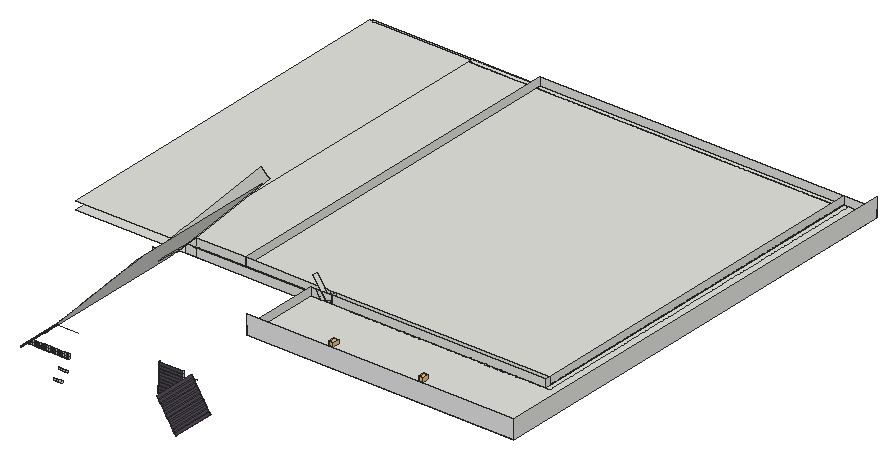
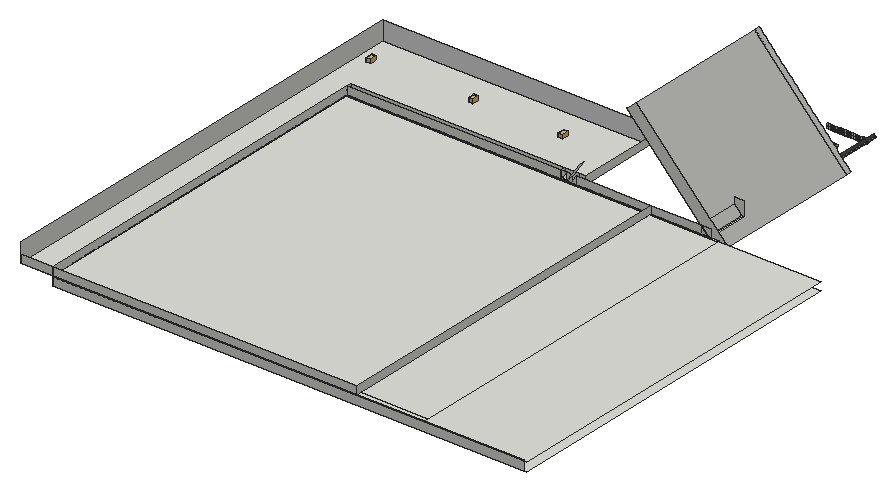
# SketchUp Ruby script. Lengths in inches.
U = 1.inch
M = Sketchup.active_model
def pt(a) = Geom::Point3d.new(a.map { |v| v * U })
def face(e, loops, mat)
  f = e.add_face(loops[0].map { |a| pt(a) })
  loops[1..].each { |l| e.add_face(l.map { |a| pt(a) }).erase! }
  f.material = f.back_material = mat if mat
  f
end
# faces: each face lists its corners as indices into pts; further lists are holes
def faces(e, pts, list, mat = nil) = list.each { |f| face(e, (f[0].is_a?(Array) ? f : [f]).map { |l| l.map { |i| pts[i] } }, mat) }
# xy, xz, yz: faces in a plane at the given z, y or x. An outline is a flat list of corners, or four numbers for a rectangle; further outlines are holes
def ring(l) = l.size == 4 ? [[l[0], l[1]], [l[2], l[1]], [l[2], l[3]], [l[0], l[3]]] : l.each_slice(2).to_a
def flat(e, list, mat, &to3) = list.each { |f| face(e, (f[0].is_a?(Array) ? f : [f]).map { |l| ring(l).map { |u, v| to3.(u, v) } }, mat) }
def xy(e, z, list, mat = nil) = flat(e, list, mat) { |x, y| [x, y, z] }
def xz(e, y, list, mat = nil) = flat(e, list, mat) { |x, z| [x, y, z] }
def yz(e, x, list, mat = nil) = flat(e, list, mat) { |y, z| [x, y, z] }
def lines(e, pts, list) = list.each { |a, b| e.add_line(pt(pts[a]), pt(pts[b])) }
# prism: a flat outline (further loops are holes) pulled along v
def prism(e, loops, v, mat = nil)
  f = face(e, loops, mat); d = Geom::Vector3d.new(v.map { |x| x * U })
  f.pushpull(f.normal.samedirection?(d) ? d.length : -d.length)
end
def box(e, o, s, mat = nil) = prism(e, [[o, [o[0] + s[0], o[1], o[2]], [o[0] + s[0], o[1] + s[1], o[2]], [o[0], o[1] + s[1], o[2]]]], [0, 0, s[2]], mat)
def at(x, y, z, deg = 0) = Geom::Transformation.translation(pt([x, y, z])) * Geom::Transformation.rotation(ORIGIN, Z_AXIS, deg.degrees)
def axes(o, x, y, z) = Geom::Transformation.new([*x, 0, *y, 0, *z, 0, *pt(o).to_a, 1])
def part(name) = M.definitions.add(name)
# library, detail: a bought-in or finely detailed component or shape, given as its bounding box
def library(name, o, s) = part(name).tap { |d| box(d.entities, o, s) }
def detail(e, o, s) = box(e.add_group.entities, o, s)
def put(e, d, t, mat = nil) = e.add_instance(d, t).tap { |i| i.material = mat if mat }
def group(e, t, mat = nil) = e.add_group.tap { |g| g.transformation = t; g.material = mat if mat }.entities
root = M.entities
M.materials.add("[Color M01]").color = [226, 226, 226]
M.materials.add("[Color M06]").color = [79, 71, 84]
c1 = library("Group\#13",[0,0,0],[3.54,3.54,3.9375])
xy(root,306.39,[[2350.98,523.75,2381.95,526.125]])
xy(root,307.2,[[2350.98,523.75,2381.95,526.125]])
xy(root,310.33,[[2350.98,523.75,2381.95,526.125]])
xy(root,311.14,[[2350.98,523.75,2381.95,526.125]])
xy(root,314.27,[[2350.98,523.75,2381.95,526.125]])
xy(root,315.08,[[2350.98,524.25,2381.95,526.125]])
xy(root,318.2,[[2350.98,524.25,2381.95,526.125]])
xy(root,319.01,[[2350.98,524.25,2381.95,526.125]])
xy(root,322.14,[[2350.98,524.25,2381.95,526.125]])
xy(root,322.89,[[2350.98,524.25,2381.95,526.125]])
xy(root,326.02,[[2350.98,524.25,2381.95,526.125]])
xy(root,326.76,[[2350.98,524.25,2381.95,526.125]])
xy(root,328,[[2079.13,732.2,2683.5,1201.875]])
xy(root,329.89,[[2350.98,524.25,2381.95,526.125]])
xy(root,330.64,[[2350.98,524.25,2381.95,526.125]])
xy(root,333.77,[[2350.98,524.25,2381.95,526.125]])
xy(root,334.51,[[2350.98,524.25,2381.95,526.125]])
xy(root,336.02,[[2220.6875,480.14,2223,480.77],[2223.6,480.14,2225.91,480.77],[2226.51,480.14,2228.82,480.77],[2229.42,480.14,2231.73,480.77],[2232.33,480.14,2234.65,480.77],
  [2235.25,480.14,2237.56,480.77],[2238.16,480.14,2240.47,480.77],[2241.07,480.14,2243.38,480.77],[2243.98,480.14,2246.29,480.77],[2246.89,480.14,2249.21,480.77],
  [2249.81,480.14,2252.12,480.77],[2252.72,480.14,2255.03,480.77],[2255.63,480.14,2257.94,480.77],[2258.54,480.14,2260.86,480.77],[2261.45,480.14,2263.77,480.77],
  [2264.37,480.14,2266.68,480.77],[2267.28,480.14,2269.59,480.77],[2270.19,480.14,2272.5,480.77]])
xy(root,336.52,[[2220.6875,480.14,2223,480.77],[2223.6,480.14,2225.91,480.77],[2226.51,480.14,2228.82,480.77],[2229.42,480.14,2231.73,480.77],[2232.33,480.14,2234.65,480.77],
  [2235.25,480.14,2237.56,480.77],[2238.16,480.14,2240.47,480.77],[2241.07,480.14,2243.38,480.77],[2243.98,480.14,2246.29,480.77],[2246.89,480.14,2249.21,480.77],
  [2249.81,480.14,2252.12,480.77],[2252.72,480.14,2255.03,480.77],[2255.63,480.14,2257.94,480.77],[2258.54,480.14,2260.86,480.77],[2261.45,480.14,2263.77,480.77],
  [2264.37,480.14,2266.68,480.77],[2267.28,480.14,2269.59,480.77],[2270.19,480.14,2272.5,480.77]])
xy(root,337.64,[[2350.98,524.25,2381.95,526.125]])
xy(root,338.39,[[2350.98,524.25,2381.95,526.125]])
xy(root,338.84,[[2222.47,480.14,2223,480.77],[2223.6,480.14,2225.91,480.77],[2226.51,480.14,2228.82,480.77],[2229.42,480.14,2231.73,480.77],[2232.33,480.14,2234.65,480.77],
  [2235.25,480.14,2237.56,480.77],[2238.16,480.14,2240.47,480.77],[2241.07,480.14,2243.38,480.77],[2243.98,480.14,2246.29,480.77],[2246.89,480.14,2249.21,480.77],
  [2249.81,480.14,2252.12,480.77],[2252.72,480.14,2255.03,480.77],[2255.63,480.14,2257.94,480.77],[2258.54,480.14,2260.86,480.77],[2261.45,480.14,2263.77,480.77],
  [2264.37,480.14,2266.68,480.77],[2267.28,480.14,2269.59,480.77],[2270.19,480.14,2272.5,480.77]])
xy(root,338.875,[[2079.13,732.2,2683.5,1201.875]])
xy(root,339.34,[[2223.6,480.14,2225.91,480.77],[2226.51,480.14,2228.82,480.77],[2229.42,480.14,2231.73,480.77],[2232.33,480.14,2234.65,480.77],[2235.25,480.14,2237.56,480.77],
  [2238.16,480.14,2240.47,480.77],[2241.07,480.14,2243.38,480.77],[2243.98,480.14,2246.29,480.77],[2246.89,480.14,2249.21,480.77],[2249.81,480.14,2252.12,480.77],
  [2252.72,480.14,2255.03,480.77],[2255.63,480.14,2257.94,480.77],[2258.54,480.14,2260.86,480.77],[2261.45,480.14,2263.77,480.77],[2264.37,480.14,2266.68,480.77],
  [2267.28,480.14,2269.59,480.77],[2270.19,480.14,2272.5,480.77]])
xy(root,340.125,[[2384.28,623.84,2384.28,726.125,2436.62,726.125,2436.62,724.8125,2442.7,724.8125,2442.7,726.125,2446.12,726.125,2446.12,724.8125,2452.2,724.8125,2452.2,726.125,2455.62,726.125,2455.62,724.8125,2461.7,724.8125,2461.7,726.125,2465.12,726.125,2465.12,724.8125,2471.2,724.8125,2471.2,726.125,2474.62,726.125,2474.62,724.8125,2480.7,724.8125,2480.7,726.125,2484.12,726.125,2484.12,724.8125,2490.2,724.8125,2490.2,726.125,2493.62,726.125,2493.62,724.8125,2499.7,724.8125,2499.7,726.125,2503.12,726.125,2503.12,724.8125,2509.2,724.8125,2509.2,726.125,2512.62,726.125,2512.62,724.8125,2518.7,724.8125,2518.7,726.125,2522.12,726.125,2522.12,724.8125,2528.2,724.8125,2528.2,726.125,2531.62,726.125,2531.62,724.8125,2537.7,724.8125,2537.7,726.125,2541.12,726.125,2541.12,724.8125,2547.2,724.8125,2547.2,726.125,2550.62,726.125,2550.62,724.8125,2556.7,724.8125,2556.7,726.125,2560.12,726.125,2560.12,724.8125,2566.2,724.8125,2566.2,726.125,2569.62,726.125,2569.62,724.8125,2575.7,724.8125,2575.7,726.125,2579.12,726.125,2579.12,724.8125,2585.2,724.8125,2585.2,726.125,2588.62,726.125,2588.62,724.8125,2594.7,724.8125,2594.7,726.125,2598.12,726.125,2598.12,724.8125,2604.2,724.8125,2604.2,726.125,2607.62,726.125,2607.62,724.8125,2613.7,724.8125,2613.7,726.125,2617.12,726.125,2617.12,724.8125,2623.2,724.8125,2623.2,726.125,2626.62,726.125,2626.62,724.8125,2632.7,724.8125,2632.7,726.125,2636.12,726.125,2636.12,724.8125,2642.2,724.8125,2642.2,726.125,2645.62,726.125,2645.62,724.8125,2651.7,724.8125,2651.7,726.125,2655.12,726.125,2655.12,724.8125,2661.2,724.8125,2661.2,726.125,2664.62,726.125,2664.62,724.8125,2670.7,724.8125,2670.7,726.125,2674.12,726.125,2674.12,724.8125,2680.2,724.8125,2680.2,726.125,2683.62,726.125,2683.62,724.8125,2689.7,724.8125,2689.7,1201.875,2724.93,1201.875,2724.93,623.84],[2219.8,678.64,2222.65,726.125],[2436.62,724.8125,2442.7,726.125],[2446.12,724.8125,2452.2,726.125],[2455.62,724.8125,2461.7,726.125],
  [2465.12,724.8125,2471.2,726.125],[2474.62,724.8125,2480.7,726.125],[2484.12,724.8125,2490.2,726.125],[2493.62,724.8125,2499.7,726.125],[2503.12,724.8125,2509.2,726.125],
  [2512.62,724.8125,2518.7,726.125],[2522.12,724.8125,2528.2,726.125],[2531.62,724.8125,2537.7,726.125],[2541.12,724.8125,2547.2,726.125],[2550.62,724.8125,2556.7,726.125],
  [2560.12,724.8125,2566.2,726.125],[2569.62,724.8125,2575.7,726.125],[2579.12,724.8125,2585.2,726.125],[2588.62,724.8125,2594.7,726.125],[2598.12,724.8125,2604.2,726.125],
  [2607.62,724.8125,2613.7,726.125],[2617.12,724.8125,2623.2,726.125],[2626.62,724.8125,2632.7,726.125],[2636.12,724.8125,2642.2,726.125],[2645.62,724.8125,2651.7,726.125],
  [2655.12,724.8125,2661.2,726.125],[2664.62,724.8125,2670.7,726.125],[2674.12,724.8125,2680.2,726.125],[2683.62,724.8125,2689.7,1201.875],[2219.8,726.125,2222.65,732.2],
  [2410.35,726.125,2683.5,732.2],[2683.5,726.125,2683.62,732.2],[2209.43,732.2,2295.55,734.4375],[2295.55,732.2,2410.35,734.4375],[2410.35,732.2,2683.5,734.4375],
  [2683.5,732.2,2683.62,734.4375],[2209.43,734.4375,2295.55,1195.68],[2295.55,734.4375,2683.5,1195.68],[2683.5,734.4375,2683.62,1195.8],[2209.43,1195.68,2295.55,1195.8],
  [2295.55,1195.68,2683.5,1195.8],[2209.43,1195.8,2295.55,1201.875],[2295.55,1195.8,2683.5,1201.875],[2683.5,1195.8,2683.62,1201.875]])
xz(root,480.64,[[2252.6875,305.35,2255,307.67],[2255.6,305.35,2257.91,307.67],[2258.51,305.35,2260.83,307.67],[2261.43,305.35,2263.74,307.67]])
xz(root,480.7,[[2258.54,319.65,2260.86,321.96],[2261.45,319.65,2263.77,321.96],[2264.37,319.65,2266.68,321.96],[2267.28,319.65,2269.59,321.96]])
xz(root,521.5625,[[2419,305.32,2419.37,305.56,2417.67,308.2,2417.3,307.97],[2416.77,308.8,2417.14,309.03,2415.44,311.68,2415.08,311.44],[2414.54,312.27,2414.91,312.51,2413.22,315.15,2412.85,314.91],[2412.32,315.74,2412.6875,315.98,2410.99,318.62,2410.625,318.38],[2410.09,319.21,2410.46,319.45,2408.77,322.09,2408.4,321.86],
  [2407.87,322.6875,2408.23,322.92,2406.54,325.57,2406.17,325.33],[2405.64,326.16,2406.01,326.4,2404.3125,329.04,2403.94,328.8],[2403.41,329.63,2403.78,329.87,2402.09,332.51,2401.72,332.28],[2401.1875,333.11,2401.55,333.34,2399.86,335.98,2399.49,335.75],[2398.96,336.58,2399.33,336.8125,2397.63,339.46,2397.27,339.22],
  [2221.68,338.19,2223.1,339.7,2222.65,340.125,2221.23,338.62],[2223.1,339.7,2223.5,340.125,2222.65,340.125],[2396.73,340.05,2397.1,340.29,2395.41,342.93,2395.04,342.69],[2222.65,340.125,2223.5,340.125,2224.11,340.76,2223.65,341.19]])
xz(root,523.75,[[2350.98,307.2,2381.95,310.33],[2350.98,311.14,2381.95,314.27]],"[Color M06]")
xz(root,524.25,[[2350.98,315.08,2381.95,318.2],[2350.98,319.01,2381.95,322.14],[2350.98,322.89,2381.95,326.02],[2350.98,326.76,2381.95,329.89],[2350.98,330.64,2381.95,333.77],
  [2350.98,334.51,2381.95,337.64],[2350.98,338.39,2381.95,341.52]],"[Color M06]")
xz(root,526.125,[[2350.98,306.39,2381.95,307.2],[2350.98,310.33,2381.95,311.14],[2350.98,314.27,2381.95,315.08],[2350.98,318.2,2381.95,319.01],[2350.98,322.14,2381.95,322.89],
  [2350.98,326.02,2381.95,326.76],[2350.98,329.89,2381.95,330.64],[2350.98,333.77,2381.95,334.51],[2350.98,337.64,2381.95,338.39]])
xz(root,623.84,[[2384.28,340.125,2724.93,363.75]],"[Color M01]")
xz(root,678.64,[[2219.8,340.125,2222.65,340.125,2232.12,350.1875,2232.12,358.5,2219.8,358.5]])
xz(root,726.125,[[2384.28,340.125,2384.28,350.1875,2390.75,350.1875,2397.21,340.125],[2397.21,340.125,2402.92,340.125,2396.47,350.1875,2390.75,350.1875],[2402.92,340.125,2396.47,350.1875,2410.35,350.1875,2410.35,340.125,2408.18,343.5],[2402.92,340.125,2408.18,343.5,2410.35,340.125],[2410.35,340.125,2683.5,350.1875]])
xz(root,731.75,[[2209.43,326.08,2198.75,336.13,2202.51,340.125,2219.08,357.73,2219.8,357.04,2219.8,358.5,2315.81,460.49,2323.34,453.39,2326.48,450.4375,2232.12,350.1875,2222.65,340.125]])
xz(root,732.2,[[2219.8,328,2232.12,328,2232.12,338.875,2221.47,338.875,2219.8,337.11],[2232.12,328,2390.75,338.875],[2390.75,328,2396.47,338.875],[2396.47,328,2403.9,328,2403.9,329.69,2398.01,338.875,2396.47,338.875],[2403.9,328,2404.98,328,2403.9,329.69],
  [2404.98,328,2410.35,328,2410.35,338.875,2403.9,338.875,2403.9,329.69],[2410.35,328,2683.5,338.875],[2403.9,329.69,2403.9,338.875,2398.01,338.875],[2219.8,338.875,2219.8,340.125,2222.65,340.125,2221.47,338.875],[2221.47,338.875,2232.12,338.875,2232.12,340.125,2222.65,340.125],
  [2232.12,338.875,2390.75,340.125],[2390.75,338.875,2396.47,340.125],[2396.47,338.875,2398.01,338.875,2397.21,340.125,2396.47,340.125],[2398.01,338.875,2403.9,338.875,2403.9,340.125,2397.21,340.125],[2403.9,338.875,2410.35,340.125],
  [2410.35,338.875,2683.5,340.125],[2219.8,340.125,2219.8,350.1875,2232.12,350.1875,2222.65,340.125],[2222.65,340.125,2232.12,350.1875,2232.12,340.125],[2232.12,340.125,2295.55,350.1875],[2295.55,340.125,2390.75,350.1875],
  [2390.75,340.125,2396.47,340.125,2396.47,341.27,2390.75,350.1875],[2396.47,340.125,2397.21,340.125,2396.47,341.27],[2397.21,340.125,2402.92,340.125,2396.47,350.1875,2396.47,341.27],[2402.92,340.125,2403.9,340.75,2403.9,350.1875,2396.47,350.1875],[2402.92,340.125,2403.9,340.125,2403.9,340.75],
  [2403.9,340.125,2410.35,340.125,2410.35,350.1875,2403.9,350.1875,2408.18,343.5,2403.9,340.75],[2410.35,340.125,2683.5,350.1875]])
xz(root,1201.875,[[2082.95,328,2683.5,338.875],[2082.95,338.875,2683.5,340.125],[2295.55,340.125,2683.5,350.1875],[2683.5,340.125,2724.93,350.1875]])
yz(root,2220.6875,[[480.14,336.52,480.77,336.93]])
yz(root,2223,[[480.14,336.52,480.77,338.84]])
yz(root,2223.6,[[480.14,336.52,480.77,338.84],[480.14,339.34,480.77,340.04]])
yz(root,2225.91,[[480.14,336.52,480.77,338.84],[480.14,339.34,480.77,341.65]])
yz(root,2226.51,[[480.14,336.52,480.77,338.84],[480.14,339.34,480.77,341.65]])
yz(root,2228.82,[[480.14,336.52,480.77,338.84],[480.14,339.34,480.77,341.65]])
yz(root,2229.42,[[480.14,336.52,480.77,338.84],[480.14,339.34,480.77,341.65]])
yz(root,2231.73,[[480.14,336.52,480.77,338.84],[480.14,339.34,480.77,341.65]])
yz(root,2232.33,[[480.14,336.52,480.77,338.84],[480.14,339.34,480.77,341.65]])
yz(root,2234.65,[[480.14,336.52,480.77,338.84],[480.14,339.34,480.77,341.65]])
yz(root,2235.25,[[480.14,336.52,480.77,338.84],[480.14,339.34,480.77,341.65]])
yz(root,2237.56,[[480.14,336.52,480.77,338.84],[480.14,339.34,480.77,341.65]])
yz(root,2238.16,[[480.14,336.52,480.77,338.84],[480.14,339.34,480.77,341.65]])
yz(root,2240.47,[[480.14,336.52,480.77,338.84],[480.14,339.34,480.77,341.65]])
yz(root,2241.07,[[480.14,336.52,480.77,338.84],[480.14,339.34,480.77,341.65]])
yz(root,2243.38,[[480.14,336.52,480.77,338.84],[480.14,339.34,480.77,341.65]])
yz(root,2243.98,[[480.14,336.52,480.77,338.84],[480.14,339.34,480.77,341.65]])
yz(root,2246.29,[[480.14,336.52,480.77,338.84],[480.14,339.34,480.77,341.65]])
yz(root,2246.89,[[480.14,336.52,480.77,338.84],[480.14,339.34,480.77,341.65]])
yz(root,2249.21,[[480.14,336.52,480.77,338.84],[480.14,339.34,480.77,341.65]])
yz(root,2249.81,[[480.14,336.52,480.77,338.84],[480.14,339.34,480.77,341.65]])
yz(root,2252.12,[[480.14,336.52,480.77,338.84],[480.14,339.34,480.77,341.65]])
yz(root,2252.72,[[480.14,336.52,480.77,338.84],[480.14,339.34,480.77,341.65]])
yz(root,2255.03,[[480.14,336.52,480.77,338.84],[480.14,339.34,480.77,341.65]])
yz(root,2255.63,[[480.14,336.52,480.77,338.84],[480.14,339.34,480.77,341.65]])
yz(root,2257.94,[[480.14,336.52,480.77,338.84],[480.14,339.34,480.77,341.65]])
yz(root,2258.54,[[480.14,336.52,480.77,338.84],[480.14,339.34,480.77,341.65]])
yz(root,2260.86,[[480.14,336.52,480.77,338.84],[480.14,339.34,480.77,341.65]])
yz(root,2261.45,[[480.14,336.52,480.77,338.84],[480.14,339.34,480.77,341.65]])
yz(root,2263.77,[[480.14,336.52,480.77,338.84],[480.14,339.34,480.77,341.65]])
yz(root,2264.37,[[480.14,336.52,480.77,338.84],[480.14,339.34,480.77,341.65]])
yz(root,2266.68,[[480.14,336.52,480.77,338.84],[480.14,339.34,480.77,341.65]])
yz(root,2267.28,[[480.14,336.52,480.77,338.84],[480.14,339.34,480.77,341.65]])
yz(root,2269.59,[[480.14,336.52,480.77,338.84],[480.14,339.34,480.77,341.65]])
yz(root,2270.19,[[480.14,336.52,480.77,338.84],[480.14,339.34,480.77,341.65]])
yz(root,2272.5,[[480.14,336.52,480.77,338.84],[480.14,339.34,480.77,341.65]])
yz(root,2295.55,[[732.2,340.125,1201.875,350.1875]])
yz(root,2350.98,[[523.75,307.2,526.125,310.33],[523.75,311.14,526.125,314.27],[524.25,315.08,526.125,318.2],[524.25,319.01,526.125,322.14],[524.25,322.89,526.125,326.02],
  [524.25,326.76,526.125,329.89],[524.25,330.64,526.125,333.77],[524.25,334.51,526.125,337.64],[524.25,338.39,526.125,341.52]])
yz(root,2381.95,[[523.75,307.2,526.125,310.33],[523.75,311.14,526.125,314.27],[524.25,315.08,526.125,318.2],[524.25,319.01,526.125,322.14],[524.25,322.89,526.125,326.02],
  [524.25,326.76,526.125,329.89],[524.25,330.64,526.125,333.77],[524.25,334.51,526.125,337.64],[524.25,338.39,526.125,341.52]])
yz(root,2384.28,[[623.84,340.125,726.125,350.1875]])
yz(root,2410.35,[[726.125,340.125,732.2,350.1875]])
yz(root,2683.5,[[732.2,328,1195.68,338.875],[1195.68,328,1201.875,338.875],[732.2,338.875,1195.68,340.125],[1195.68,338.875,1201.875,340.125],[726.125,340.125,732.2,350.1875],
  [732.2,340.125,1201.875,350.1875]])
yz(root,2724.93,[[623.84,340.125,1201.875,363.75]])
p = [[2417.3,521.5625,307.97],[2419,521.5625,305.32],[2419,467.1875,305.32],[2417.3,467.1875,307.97],[2419.37,521.5625,305.56],[2419.37,467.1875,305.56],
  [2417.67,467.1875,308.2],[2417.67,521.5625,308.2],[2417.14,467.1875,309.03],[2417.14,521.5625,309.03],[2415.08,521.5625,311.44],[2416.77,521.5625,308.8],
  [2416.77,467.1875,308.8],[2415.08,467.1875,311.44],[2415.44,467.1875,311.68],[2415.44,521.5625,311.68],[2414.91,467.1875,312.51],[2414.91,521.5625,312.51],
  [2412.85,521.5625,314.91],[2414.54,521.5625,312.27],[2414.54,467.1875,312.27],[2412.85,467.1875,314.91],[2413.22,467.1875,315.15],[2413.22,521.5625,315.15],
  [2412.6875,467.1875,315.98],[2412.6875,521.5625,315.98],[2410.625,521.5625,318.38],[2412.32,521.5625,315.74],[2412.32,467.1875,315.74],[2410.625,467.1875,318.38],
  [2410.99,467.1875,318.62],[2410.99,521.5625,318.62],[2410.46,467.1875,319.45],[2410.46,521.5625,319.45],[2408.4,521.5625,321.86],[2410.09,521.5625,319.21],
  [2410.09,467.1875,319.21],[2408.4,467.1875,321.86],[2408.77,467.1875,322.09],[2408.77,521.5625,322.09],[2408.23,467.1875,322.92],[2408.23,521.5625,322.92],
  [2406.17,521.5625,325.33],[2407.87,521.5625,322.6875],[2407.87,467.1875,322.6875],[2406.17,467.1875,325.33],[2406.54,467.1875,325.57],[2406.54,521.5625,325.57],
  [2406.01,467.1875,326.4],[2406.01,521.5625,326.4],[2209.43,528.48,326.08],[2326.48,528.48,450.4375],[2326.48,521.5625,450.4375],[2326.17,521.5625,450.11],
  [2325.9,521.5625,449.82],[2323.48,521.5625,447.25],[2322.61,521.5625,446.32],[2320.19,521.5625,443.75],[2319.31,521.5625,442.8125],[2316.89,521.5625,440.24],
  [2316.01,521.5625,439.31],[2313.59,521.5625,436.74],[2312.71,521.5625,435.81],[2310.29,521.5625,433.23],[2309.41,521.5625,432.3],[2306.99,521.5625,429.73],
  [2306.11,521.5625,428.8],[2303.69,521.5625,426.23],[2302.81,521.5625,425.29],[2300.39,521.5625,422.72],[2299.52,521.5625,421.79],[2297.1,521.5625,419.22],
  [2296.22,521.5625,418.28],[2293.8,521.5625,415.71],[2292.92,521.5625,414.78],[2290.5,521.5625,412.21],[2289.62,521.5625,411.28],[2287.2,521.5625,408.7],
  [2286.32,521.5625,407.77],[2283.9,521.5625,405.2],[2283.02,521.5625,404.27],[2280.6,521.5625,401.7],[2279.73,521.5625,400.76],[2277.3,521.5625,398.19],
  [2276.43,521.5625,397.26],[2274.01,521.5625,394.6875],[2273.13,521.5625,393.75],[2270.71,521.5625,391.18],[2269.83,521.5625,390.25],[2267.41,521.5625,387.68],
  [2266.53,521.5625,386.75],[2264.11,521.5625,384.17],[2263.23,521.5625,383.24],[2260.8125,521.5625,380.67],[2259.93,521.5625,379.74],[2257.51,521.5625,377.17],
  [2256.64,521.5625,376.23],[2254.21,521.5625,373.66],[2253.34,521.5625,372.73],[2250.92,521.5625,370.16],[2250.04,521.5625,369.23],[2247.62,521.5625,366.65],
  [2246.74,521.5625,365.72],[2244.32,521.5625,363.15],[2243.44,521.5625,362.22],[2241.02,521.5625,359.64],[2240.14,521.5625,358.71],[2237.72,521.5625,356.14],
  [2236.84,521.5625,355.21],[2234.42,521.5625,352.64],[2233.55,521.5625,351.7],[2231.125,521.5625,349.13],[2230.25,521.5625,348.2],[2227.83,521.5625,345.63],
  [2226.95,521.5625,344.7],[2224.53,521.5625,342.125],[2223.65,521.5625,341.19],[2222.65,521.5625,340.125],[2221.23,521.5625,338.62],[2220.35,521.5625,337.6875],
  [2217.93,521.5625,335.11],[2217.05,521.5625,334.18],[2214.63,521.5625,331.61],[2213.75,521.5625,330.68],[2211.33,521.5625,328.11],[2210.46,521.5625,327.17],
  [2209.43,521.5625,326.08],[2209.43,719.59,326.08],[2222.65,719.59,340.125],[2222.65,678.64,340.125],[2232.12,678.64,350.1875],[2232.12,719.59,350.1875],
  [2326.48,719.59,450.4375],[2209.43,719.2,326.08],[2403.94,521.5625,328.8],[2405.64,521.5625,326.16],[2405.64,467.1875,326.16],[2403.94,467.1875,328.8],
  [2404.3125,467.1875,329.04],[2404.3125,521.5625,329.04],[2403.78,467.1875,329.87],[2403.78,521.5625,329.87],[2401.72,521.5625,332.28],[2403.41,521.5625,329.63],
  [2403.41,467.1875,329.63],[2401.72,467.1875,332.28],[2402.09,467.1875,332.51],[2402.09,521.5625,332.51],[2401.55,467.1875,333.34],[2401.55,521.5625,333.34],
  [2399.49,521.5625,335.75],[2401.1875,521.5625,333.11],[2401.1875,467.1875,333.11],[2399.49,467.1875,335.75],[2399.86,467.1875,335.98],[2399.86,521.5625,335.98],
  [2399.33,467.1875,336.8125],[2399.33,521.5625,336.8125],[2397.27,521.5625,339.22],[2398.96,521.5625,336.58],[2398.96,467.1875,336.58],[2397.27,467.1875,339.22],
  [2222.47,480.14,338.84],[2220.6875,480.14,336.93],[2220.6875,480.77,336.93],[2222.47,480.77,338.84],[2221.23,467.1875,338.62],[2220.35,467.1875,337.6875],
  [2221.68,521.5625,338.19],[2221.68,467.1875,338.19],[2223.5,521.5625,340.125],[2224.11,521.5625,340.76],[2224.11,467.1875,340.76],[2223.1,521.5625,339.7],
  [2397.63,467.1875,339.46],[2397.63,521.5625,339.46],[2397.1,467.1875,340.29],[2397.1,521.5625,340.29],[2397.21,521.5625,340.125],[2225.11,480.14,341.65],
  [2223.6,480.14,340.04],[2223.6,480.77,340.04],[2225.11,480.77,341.65],[2395.04,521.5625,342.69],[2396.73,521.5625,340.05],[2396.73,467.1875,340.05],
  [2395.04,467.1875,342.69],[2232.12,731.75,350.1875],[2222.65,731.75,340.125],[2222.65,726.125,340.125],[2387.78,726.125,363.75],[2387.01,726.125,364.9375],
  [2387.01,732.2,364.9375],[2396.47,732.2,350.1875],[2402.92,732.2,340.125],[2402.92,726.125,340.125],[2396.47,726.125,350.1875],[2390.75,726.125,359.1],
  [2408.18,726.125,343.5],[2403.9,732.2,340.75],[2408.18,732.2,343.5],[2222.65,732.2,340.125],[2232.12,732.2,350.1875],[2251.48,521.5625,340.125],
  [2402.92,521.5625,340.125]]
faces(root,p,[[0,1,2,3],[6,8,9,7],[10,11,12,13],[14,16,17,15],[18,19,20,21],[22,24,25,23],[26,27,28,29],[30,32,33,31],
  [34,35,36,37],[38,40,41,39],[42,43,44,45],[46,48,49,47],[134,135,136,137],[138,140,141,139],[142,143,144,145],[146,148,149,147],
  [150,151,152,153],[154,156,157,155],[158,159,160,161],[119,118,166,167],[170,171,172,169,168,173],[174,176,177,178,175],[183,184,185,186]],"[Color M06]")
faces(root,p,[[4,5,2,1],[6,7,0,3],[9,8,12,11],[14,15,10,13],[17,16,20,19],[22,23,18,21],[25,24,28,27],[30,31,26,29],
  [33,32,36,35],[38,39,34,37],[41,40,44,43],[46,47,42,45],[50,51,52,53,54,55,56,57,58,59,60,61,62,63,64,65,66,67,68,69,70,71,72,73,74,75,76,77,78,79,80,81,82,83,84,85,86,87,88,89,90,91,92,93,94,95,96,97,98,99,100,101,102,103,104,105,106,107,108,109,110,111,112,113,114,115,116,117,118,119,120,121,122,123,124,125,126],[127,128,129,130,131,132,51,50,133],[49,48,136,135],[138,139,134,137],
  [141,140,144,143],[146,147,142,145],[149,148,152,151],[154,155,150,153],[157,156,160,159],[162,163,164,165],[166,118,168,169],[174,175,158,161],
  [179,180,181,182],[177,176,185,184],[128,131,130,129],[128,131,187,188,189],[190,191,192,193,194,195,196,197],[198,195,194,199,200],[187,188,201,202]])
lines(root,p,[[203,170],[178,204]])
put(root,c1,axes([2466.33,658.52,344.6875],[-1.5535,0,0],[0,2.39,0],[0,0,-3.63878]))
put(root,c1,axes([2580.89,658.52,344.6875],[-1.5535,0,0],[0,2.39,0],[0,0,-3.63878]))
put(root,c1,axes([2711.45,658.52,344.6875],[-1.5535,0,0],[0,2.39,0],[0,0,-3.63878]))
